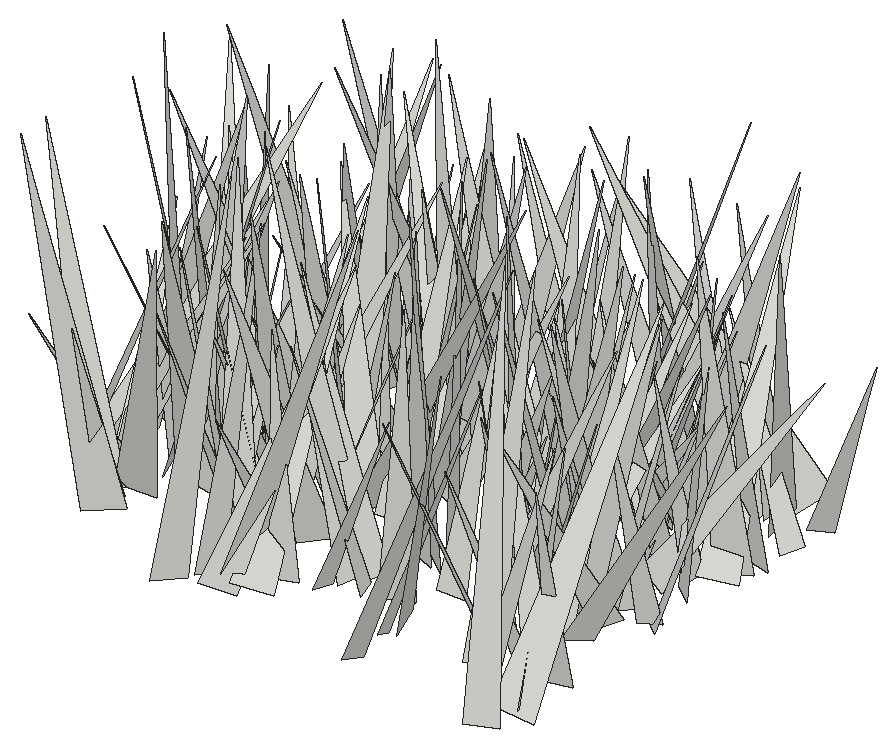
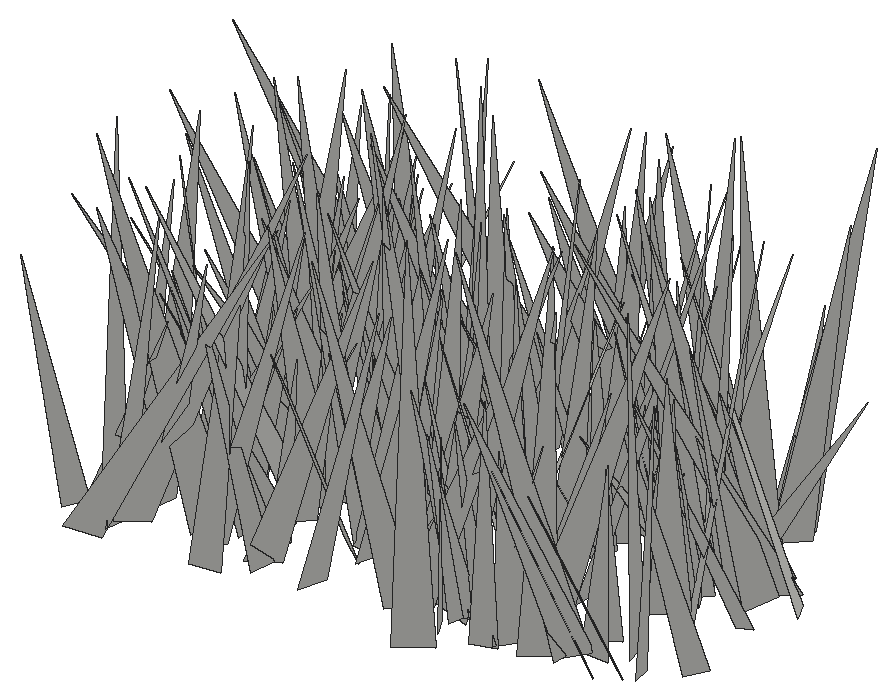
# SketchUp Ruby script. Lengths in inches.
U = 1.inch
M = Sketchup.active_model
def pt(a) = Geom::Point3d.new(a.map { |v| v * U })
def face(e, loops, mat)
  f = e.add_face(loops[0].map { |a| pt(a) })
  loops[1..].each { |l| e.add_face(l.map { |a| pt(a) }).erase! }
  f.material = f.back_material = mat if mat
  f
end
# faces: each face lists its corners as indices into pts; further lists are holes
def faces(e, pts, list, mat = nil) = list.each { |f| face(e, (f[0].is_a?(Array) ? f : [f]).map { |l| l.map { |i| pts[i] } }, mat) }
# xy, xz, yz: faces in a plane at the given z, y or x. An outline is a flat list of corners, or four numbers for a rectangle; further outlines are holes
def ring(l) = l.size == 4 ? [[l[0], l[1]], [l[2], l[1]], [l[2], l[3]], [l[0], l[3]]] : l.each_slice(2).to_a
def flat(e, list, mat, &to3) = list.each { |f| face(e, (f[0].is_a?(Array) ? f : [f]).map { |l| ring(l).map { |u, v| to3.(u, v) } }, mat) }
def xy(e, z, list, mat = nil) = flat(e, list, mat) { |x, y| [x, y, z] }
def xz(e, y, list, mat = nil) = flat(e, list, mat) { |x, z| [x, y, z] }
def yz(e, x, list, mat = nil) = flat(e, list, mat) { |y, z| [x, y, z] }
def lines(e, pts, list) = list.each { |a, b| e.add_line(pt(pts[a]), pt(pts[b])) }
# prism: a flat outline (further loops are holes) pulled along v
def prism(e, loops, v, mat = nil)
  f = face(e, loops, mat); d = Geom::Vector3d.new(v.map { |x| x * U })
  f.pushpull(f.normal.samedirection?(d) ? d.length : -d.length)
end
def box(e, o, s, mat = nil) = prism(e, [[o, [o[0] + s[0], o[1], o[2]], [o[0] + s[0], o[1] + s[1], o[2]], [o[0], o[1] + s[1], o[2]]]], [0, 0, s[2]], mat)
def at(x, y, z, deg = 0) = Geom::Transformation.translation(pt([x, y, z])) * Geom::Transformation.rotation(ORIGIN, Z_AXIS, deg.degrees)
def axes(o, x, y, z) = Geom::Transformation.new([*x, 0, *y, 0, *z, 0, *pt(o).to_a, 1])
def part(name) = M.definitions.add(name)
# library, detail: a bought-in or finely detailed component or shape, given as its bounding box
def library(name, o, s) = part(name).tap { |d| box(d.entities, o, s) }
def detail(e, o, s) = box(e.add_group.entities, o, s)
def put(e, d, t, mat = nil) = e.add_instance(d, t).tap { |i| i.material = mat if mat }
def group(e, t, mat = nil) = e.add_group.tap { |g| g.transformation = t; g.material = mat if mat }.entities
root = M.entities
c1 = part("fur_instance\#9")
p = [[0.8125,0,1.79],[0.67,-0.02,1.48],[0,-0.11,0],[0,0.11,0]]
faces(c1.entities,p,[[0,1,2,3]])
put(root,c1,axes([156.88,414.5625,-27.1],[4.55494,-1.38322,1.77977],[-1.90749,-4.50337,1.38185],[-1.20098,1.9065,4.55536]))
put(root,c1,axes([138.06,416.81,-27.1],[2.50523,-6.92108,2.84903],[-7.08461,-3.16179,-1.45116],[-2.41383,2.09672,7.21607]))
put(root,c1,axes([158.23,412.92,-27.1],[0.30584,8.28043,0.48557],[7.987,-0.4251,2.21855],[-2.2381,-0.38549,7.98355]))
put(root,c1,axes([151.5,417.05,-27.1],[6.22131,1.299,1.34326],[1.60809,-6.10017,-1.54868],[-0.95174,-1.81575,6.1639]))
put(root,c1,axes([158.52,416.99,-27.1],[1.07632,-4.38935,0.89904],[-4.4763,-1.09335,0.02097],[-0.19334,0.87825,4.51934]))
put(root,c1,axes([143.01,414.3,-27.1],[-6.71814,2.72987,2.53139],[2.23652,7.13443,-1.75826],[2.97626,0.8008,7.03521]))
put(root,c1,axes([155.51,417.1,-27.1],[-3.79986,-3.34827,0.10157],[-3.34083,3.7767,-0.4853],[-0.24505,0.43103,5.04126]))
put(root,c1,axes([137.81,417.57,-27.1],[2.72704,-3.27265,0.76108],[-3.17295,-2.83078,-0.80329],[-1.10537,0.05182,4.1835]))
put(root,c1,axes([138.07,418.58,-27.1],[2.36593,-6.95857,0.28973],[-6.83072,-2.25873,1.53056],[1.359,0.76137,7.18865]))
put(root,c1,axes([156.9,417.11,-27.1],[-0.5806,-4.0301,0.94816],[-3.96701,0.26756,-1.29192],[-1.18471,1.07913,3.86131]))
put(root,c1,axes([158.72,414.83,-27.1],[-4.5247,0.14497,1.56827],[-0.47946,4.4174,-1.79167],[1.5002,1.84904,4.15738]))
put(root,c1,axes([146.21,416.8,-27.1],[-1.45922,4.42701,2.15741],[4.90506,1.50733,0.22462],[0.43952,-2.12407,4.65589]))
put(root,c1,axes([144.89,415.73,-27.1],[7.47756,-1.51643,1.55812],[-1.8154,-7.42558,1.48539],[-1.19651,1.78955,7.48379]))
put(root,c1,axes([144.78,414.83,-27.1],[-3.66435,5.27166,1.90181],[4.6134,4.12758,-2.55233],[3.18179,0.08644,5.89097]))
put(root,c1,axes([151.63,413.93,-27.1],[7.3603,1.92647,1.4977],[1.22652,-7.03518,3.02165],[-2.10951,2.63124,6.98247]))
put(root,c1,axes([144.33,418.89,-27.1],[1.81992,-3.21241,0.00061],[-3.09433,-1.75321,-0.99152],[-0.86298,-0.48823,3.55649]))
put(root,c1,axes([143.84,415.58,-27.1],[-6.0255,1.4926,2.28597],[0.94971,6.33899,-1.63567],[2.5596,1.16168,5.98825]))
put(root,c1,axes([147.59,417.28,-27.1],[4.04534,-0.8517,0.30361],[-0.87788,-4.03293,0.38361],[-0.21657,0.43867,4.11619]))
put(root,c1,axes([158.59,414.24,-27.1],[-1.16046,8.00046,0.20395],[7.87345,1.17823,-1.41992],[1.43448,0.00519,7.95851]))
put(root,c1,axes([148.91,418.0625,-27.1],[-4.66141,-1.64687,0.68606],[-1.65466,4.70851,0.06011],[0.66704,0.1713,4.94341]))
put(root,c1,axes([145.32,419.77,-27.1],[2.99002,-5.93259,1.12286],[-5.76165,-3.17812,-1.449],[-1.8055,0.31717,6.48354]))
put(root,c1,axes([141.33,419.81,-27.1],[-4.0085,-3.44331,0.94309],[-3.06456,4.04605,1.74695],[1.83147,-0.76613,4.98725]))
put(root,c1,axes([150.23,418.15,-27.1],[2.8988,-5.16102,2.16058],[-5.5292,-3.01461,0.21733],[-0.85564,1.9958,5.91539]))
put(root,c1,axes([144.27,416.76,-27.1],[-5.43034,-1.89464,0.64767],[-1.9986,5.01546,-2.08529],[-0.12137,2.18018,5.36002]))
put(root,c1,axes([137.33,417.82,-27.1],[-5.93712,3.87569,1.72238],[4.1151,5.9813,0.72589],[1.02637,-1.56207,7.0529]))
put(root,c1,axes([151.37,415.99,-27.1],[4.47299,1.54799,0.88013],[1.09405,-4.26651,1.94385],[-1.40498,1.60599,4.31572]))
put(root,c1,axes([138.91,421.1,-27.1],[6.44625,-4.17663,0.34492],[-3.99481,-6.31514,-1.81045],[-1.26676,-1.33867,7.46462]))
put(root,c1,axes([137.73,419.21,-27.1],[-0.38653,-3.78857,0.47263],[-3.40937,0.1287,-1.7566],[-1.71837,0.59684,3.37891]))
put(root,c1,axes([155.375,416.58,-27.1],[-6.19625,3.45387,1.64148],[3.0912,6.3638,-1.72156],[2.25127,0.76815,6.88178]))
put(root,c1,axes([155.24,418.5625,-27.1],[-4.18009,-2.38384,1.39005],[-2.61185,4.23208,-0.59649],[0.8906,1.22265,4.77494]))
put(root,c1,axes([143.08,418.08,-27.1],[-2.11891,6.73628,2.3501],[7.12334,2.13432,0.30482],[0.39806,-2.33612,7.05509]))
put(root,c1,axes([143.9,418.87,-27.1],[-3.99562,-4.42007,1.47298],[-4.65768,3.83659,-1.12173],[0.11293,1.84803,5.85182]))
put(root,c1,axes([142.59,418.15,-27.1],[-0.05946,3.80591,1.08242],[3.88392,0.26301,-0.71143],[0.75616,-1.05166,3.7393]))
put(root,c1,axes([145.18,416.88,-27.1],[5.43487,-1.88004,3.06705],[-2.9758,-5.47185,1.91904],[-2.02138,3.00059,5.42123]))
put(root,c1,axes([148.13,418.53,-27.1],[-8.02945,1.44749,0.94959],[1.4539,8.08421,-0.0293],[0.93976,-0.13944,8.15883]))
put(root,c1,axes([154.01,420.71,-27.1],[0.47232,-5.02453,0.37853],[-5.03579,-0.45765,0.20889],[0.17316,0.39615,5.04235]))
put(root,c1,axes([156.79,417.9375,-27.1],[-1.63602,4.97918,0.62205],[4.87533,1.42244,1.43652],[-1.18757,-1.0199,5.04036]))
put(root,c1,axes([157.19,421.46,-27.1],[2.87484,-4.36178,0.57915],[-3.91954,-2.85297,-2.03053],[-1.99945,-0.67874,4.81319]))
put(root,c1,axes([145.75,415.57,-27.1],[-4.59589,5.78444,0.11594],[5.4804,4.40003,-2.28044],[1.8543,1.33244,7.02721]))
put(root,c1,axes([143.55,420.53,-27.1],[-0.33962,-4.53633,0.58104],[-4.49375,0.22275,-0.88758],[-0.84975,0.63509,4.46159]))
put(root,c1,axes([142.36,421.87,-27.1],[6.58115,-3.41587,1.26301],[-3.10443,-6.62563,-1.74311],[-1.90417,-1.00387,7.20703]))
put(root,c1,axes([148.61,419.01,-27.1],[-5.80532,1.01557,0.17125],[1.00882,5.80466,-0.22508],[0.20737,0.19232,5.88918]))
put(root,c1,axes([138.62,422.5625,-27.1],[-3.25593,-5.45811,0.05054],[-5.36708,3.21208,1.12765],[0.99394,-0.53501,6.25464]))
put(root,c1,axes([149.46,421.22,-27.1],[-3.95013,-6.45103,2.53754],[-6.55598,4.42551,1.04517],[2.25256,1.56763,7.49179]))
put(root,c1,axes([153.51,419.5,-27.1],[2.52048,5.79703,1.2985],[5.75928,-2.03853,-2.07834],[1.45681,-1.97061,5.96983]))
put(root,c1,axes([135.79,419.68,-27.1],[4.10268,4.53992,0.30052],[4.35228,-3.79801,-2.04106],[1.3262,-1.58032,5.76861]))
put(root,c1,axes([142.4,420.125,-27.1],[-2.65775,-2.55388,1.91088],[-2.80676,3.05414,0.17806],[1.51521,1.17784,3.68161]))
put(root,c1,axes([148.78,421.14,-27.1],[-1.6159,-6.90986,2.38073],[-7.13771,2.01606,1.00679],[1.57067,2.05292,7.0245]))
put(root,c1,axes([137.93,421.52,-27.1],[3.7662,-3.06911,1.25827],[-2.92554,-3.97067,-0.92842],[-1.56328,0.03677,4.76883]))
put(root,c1,axes([151.5,419.65,-27.1],[-0.63443,5.02312,1.44392],[5.17666,0.80438,-0.52377],[0.72032,-1.3566,5.03586]))
put(root,c1,axes([157.02,419.89,-27.1],[5.8068,-2.41673,0.19711],[-2.36119,-5.5195,1.88633],[0.55156,1.81463,6.0001]))
put(root,c1,axes([136.15,420.29,-27.1],[3.52755,5.08967,0.59914],[4.90233,-3.13928,-2.19532],[1.49362,-1.71683,5.79042]))
put(root,c1,axes([139.86,420.15,-27.1],[1.56528,5.39191,1.82425],[5.61252,-1.77733,0.43748],[-0.9488,-1.61836,5.59744]))
put(root,c1,axes([155.9,421.4,-27.1],[-2.90009,-5.61636,1.60668],[-5.82709,2.65472,-1.23809],[-0.41218,1.98605,6.19848]))
put(root,c1,axes([153.88,421.9375,-27.1],[4.89387,1.35478,0.49174],[1.44124,-4.60961,-1.64362],[-0.00784,-1.71558,4.80457]))
put(root,c1,axes([146.14,420.9,-27.1],[3.85266,4.81198,3.39076],[5.17881,-4.69725,0.78179],[-2.79863,-2.06788,6.11449]))
put(root,c1,axes([155.28,423.59,-27.1],[3.26606,-6.16963,0.62937],[-6.14796,-3.31446,-0.58694],[-0.81426,0.27855,6.95607]))
put(root,c1,axes([138.24,423.05,-27.1],[-6.05203,-3.65216,2.90127],[-3.20675,6.70926,1.75646],[3.38709,-0.1736,6.84691]))
put(root,c1,axes([142.83,423.29,-27.1],[-3.8372,-2.33717,0.79383],[-2.01321,3.81242,1.493],[1.42812,-0.90538,4.23762]))
put(root,c1,axes([153.32,421.24,-27.1],[-6.66859,-2.01923,2.71074],[-2.32845,7.09045,-0.44648],[2.45024,1.24248,6.95328]))
put(root,c1,axes([158.25,422.43,-27.1],[1.30026,-4.12004,1.09762],[-4.18224,-1.45572,-0.50983],[-0.82967,0.8811,4.29016]))
put(root,c1,axes([136.82,419.54,-27.1],[-2.17484,4.53028,0.06229],[4.50087,2.16823,-0.54601],[0.51907,0.1805,4.99552]))
put(root,c1,axes([133.94,421.53,-27.1],[5.98281,3.47845,0.55141],[3.51313,-5.81778,-1.41742],[0.2481,-1.50052,6.77381]))
put(root,c1,axes([137.92,420.65,-27.1],[6.78168,2.91502,1.19431],[2.8839,-6.88568,0.43057],[-1.26762,-0.07012,7.36906]))
put(root,c1,axes([155.07,423.51,-27.1],[1.17594,-4.92519,0.34785],[-4.93492,-1.18388,-0.07952],[-0.1583,0.31979,5.06301]))
put(root,c1,axes([139.65,421.64,-27.1],[3.10895,3.01642,1.49943],[3.22004,-3.26039,-0.11754],[-0.98914,-1.13301,4.33019]))
put(root,c1,axes([151.19,422.47,-27.1],[2.68666,-2.71893,0.01615],[-2.65256,-2.616,0.85524],[0.59729,0.61233,3.72549]))
put(root,c1,axes([153.03,421.77,-27.1],[3.30994,1.56111,0.94089],[1.62723,-3.40964,-0.0672],[-0.82125,-0.46405,3.659]))
put(root,c1,axes([140.05,421.42,-27.1],[3.54809,3.00738,1.07129],[3.07779,-3.64774,0.04651],[-0.84804,-0.65624,4.65093]))
put(root,c1,axes([142.13,422.45,-27.1],[2.86459,-3.18276,1.27512],[-3.34476,-2.95943,0.1272],[-0.754,1.03614,4.28015]))
put(root,c1,axes([153.55,422.21,-27.1],[-3.32572,-4.76152,1.64129],[-5.0351,3.09772,-1.21581],[-0.11678,2.03921,5.67929]))
put(root,c1,axes([141.63,420.7,-27.1],[-0.67642,4.08917,0.12939],[3.98053,0.62749,0.97839],[-0.94522,-0.2838,4.0276]))
put(root,c1,axes([137.56,422.21,-27.1],[3.65064,-1.60023,0.53489],[-1.66152,-3.63138,0.47591],[-0.29361,0.65299,3.95745]))
put(root,c1,axes([142.9,421.66,-27.1],[0.16923,4.07191,1.2027],[4.12697,0.12503,-1.00402],[0.99752,-1.2081,3.94982]))
put(root,c1,axes([155.28,422.42,-27.1],[0.56131,-6.10589,2.64479],[-6.41112,0.21442,1.85565],[1.78167,2.69518,5.8441]))
put(root,c1,axes([138.05,421.36,-27.1],[3.6249,6.4726,3.15784],[6.5149,-4.45394,1.65071],[-3.06961,-1.8095,7.23254]))
put(root,c1,axes([156,420.01,-27.1],[0.77683,6.56918,0.32302],[6.56801,-0.79193,0.30978],[-0.34589,-0.28401,6.60769]))
put(root,c1,axes([157.04,422.73,-27.1],[-1.11932,5.12608,2.18052],[5.30702,0.30525,2.00664],[-1.6932,-2.43194,4.84799]))
put(root,c1,axes([135.375,422.09,-27.1],[6.77248,-2.83159,1.61361],[-3.13932,-6.6674,1.47599],[-0.87537,2.00399,7.19067]))
put(root,c1,axes([137.61,423.14,-27.1],[5.01911,-5.50348,2.14134],[-5.83765,-5.04831,0.7082],[-0.89193,2.07156,7.41473]))
put(root,c1,axes([140.43,425.61,-27.1],[-7.65526,-2.65251,1.50577],[-2.23878,7.64939,2.09305],[2.07148,-1.53532,7.82675]))
put(root,c1,axes([136.4,424.68,-27.1],[-5.36571,-5.00333,1.81378],[-4.95811,5.63559,0.87824],[1.93398,0.5664,7.28374]))
put(root,c1,axes([145.28,422.62,-27.1],[7.55011,-1.58138,0.22082],[-1.59514,-7.42262,1.38345],[0.0711,1.39915,7.58887]))
put(root,c1,axes([135.15,420.88,-27.1],[0.81957,8.13408,0.73803],[7.68253,-0.51597,-2.84467],[2.77248,-0.97476,7.66439]))
put(root,c1,axes([152.63,424.03,-27.1],[7.05562,-2.47543,1.6862],[-2.53392,-7.23407,-0.01726],[-1.59697,0.54154,7.47725]))
put(root,c1,axes([152.8,424.64,-27.1],[2.44609,-6.94499,1.47158],[-6.99231,-2.08787,1.76924],[1.22722,1.94671,7.14745]))
put(root,c1,axes([152.75,420.76,-27.1],[1.27817,7.72916,0.81529],[7.27012,-1.48113,2.64386],[-2.74773,-0.32349,7.37453]))
put(root,c1,axes([149.71,421.92,-27.1],[-6.21182,-1.68937,2.27799],[-2.42044,6.01654,-2.13837],[1.47806,2.75267,6.07191]))
put(root,c1,axes([135.25,423.45,-27.1],[2.3418,4.95634,1.60959],[5.19702,-2.35112,-0.32146],[-0.38351,-1.59595,5.4723]))
put(root,c1,axes([141.39,425.84,-27.1],[5.68928,-3.36377,1.44998],[-3.11585,-5.85243,-1.35122],[-1.92583,-0.46842,6.46971]))
put(root,c1,axes([147.45,421.84,-27.1],[5.41894,2.39891,1.8987],[1.67708,-5.5593,2.23748],[-2.55876,1.4367,5.48756]))
put(root,c1,axes([154.06,422.74,-27.1],[2.83544,5.2975,1.05869],[5.3487,-2.92083,0.29014],[-0.75876,-0.79328,6.00159]))
put(root,c1,axes([138.41,422.25,-27.1],[3.83996,1.68055,0.1423],[1.49178,-3.54944,1.66307],[-0.78682,1.47206,3.84756]))
put(root,c1,axes([146.5625,422.59,-27.1],[-1.26821,6.79621,1.34265],[6.86908,1.41065,-0.65215],[0.89826,-1.19212,6.8827]))
put(root,c1,axes([156.75,422.13,-27.1],[2.63197,4.07891,0.20518],[3.86496,-2.5665,1.44292],[-1.31973,0.61842,4.63495]))
put(root,c1,axes([138.45,423.51,-27.1],[-1.05429,4.67357,0.99792],[4.75005,0.91265,0.74413],[-0.52453,-1.12891,4.73287]))
put(root,c1,axes([137.33,422.9,-27.1],[3.31155,2.43431,1.59522],[1.82743,-3.61986,1.73033],[-2.2652,0.63849,3.72802]))
put(root,c1,axes([134.72,423.6875,-27.1],[1.36791,4.73736,0.76135],[4.55305,-1.0318,-1.76027],[1.51392,-1.17738,4.60599]))
put(root,c1,axes([152.19,423.78,-27.1],[3.72107,-3.56028,1.90501],[-4.03778,-3.30047,1.71878],[-0.03061,2.5656,4.85467]))
put(root,c1,axes([153.92,424.24,-27.1],[-4.56501,-1.69942,1.47091],[-1.97129,4.62695,-0.77219],[1.07964,1.26263,4.80947]))
put(root,c1,axes([149.29,425.37,-27.1],[1.54528,-3.8993,0.59524],[-3.77652,-1.27799,1.43226],[1.13873,1.05307,3.94222]))
put(root,c1,axes([158.62,422.13,-27.1],[3.88995,3.95886,0.07672],[3.75671,-3.72392,1.68217],[-1.25122,1.12695,5.2891]))
put(root,c1,axes([146.85,424.81,-27.1],[7.17764,0.6661,2.04171],[0.73913,-7.45363,-0.1667],[-2.01642,-0.36113,7.20655]))
put(root,c1,axes([147.49,424.7,-27.1],[1.43912,5.66343,2.07225],[5.60003,-0.46439,-2.61988],[2.23794,-2.47985,5.22319]))
put(root,c1,axes([155.02,425.85,-27.1],[-0.84306,-4.44176,0.86686],[-4.52258,0.85891,0.00263],[0.16427,0.85115,4.52106]))
put(root,c1,axes([154.27,422.73,-27.1],[-0.54715,4.89077,0.10405],[4.53126,0.54616,-1.84371],[1.84341,0.10915,4.56287]))
put(root,c1,axes([156.3125,425.86,-27.1],[0.08099,-5.17118,1.20761],[-5.27072,-0.22549,-0.61212],[-0.64729,1.18913,5.13546]))
put(root,c1,axes([143.2,423.86,-27.1],[3.15167,2.15202,0.19961],[2.1362,-3.1554,0.29004],[-0.32814,0.12762,3.80527]))
put(root,c1,axes([148.56,427.7,-27.1],[-2.04467,-7.63412,0.65301],[-7.56547,2.11851,1.07815],[1.21235,0.345,7.82931]))
put(root,c1,axes([152.45,426.04,-27.1],[-1.50167,-7.67594,2.08534],[-7.92089,1.24921,-1.10571],[-0.72669,2.24569,7.7429]))
put(root,c1,axes([142.38,427.95,-27.1],[-4.33714,-4.09832,0.0827],[-3.81397,4.0787,2.10515],[1.50223,-1.4771,5.58349]))
put(root,c1,axes([143.84,424.31,-27.1],[-4.18107,4.06515,1.12452],[4.17237,4.21812,0.26475],[0.61747,-0.97641,5.82552]))
put(root,c1,axes([157.47,425.88,-27.1],[-4.17455,0.44699,1.70239],[0.80041,4.38471,0.81146],[1.56757,-1.04848,4.11925]))
put(root,c1,axes([154.5,425.29,-27.1],[-3.00148,-2.27694,0.1564],[-2.20162,2.82047,-1.1898],[-0.60148,1.03841,3.57459]))
put(root,c1,axes([153.21,425.66,-27.1],[6.75875,-1.16964,0.00047],[-1.16859,-6.75255,0.29358],[0.0496,0.28936,6.85293]))
put(root,c1,axes([142.48,425.71,-27.1],[2.08402,3.38406,1.47593],[3.68931,-1.84524,-0.97848],[0.13865,-1.76538,3.85196]))
put(root,c1,axes([151.42,425.42,-27.1],[-2.68831,3.38264,1.06218],[3.54497,2.54168,0.8778],[-0.06058,-1.37662,4.23069]))
put(root,c1,axes([141.0625,423.7,-27.1],[2.76171,5.55128,0.00194],[5.48471,-2.72826,-0.95829],[0.85713,-0.42855,6.1258]))
put(root,c1,axes([157.875,424.77,-27.1],[3.73887,4.62596,1.90486],[4.75099,-4.02818,0.45718],[-1.5672,-1.17533,5.9304]))
put(root,c1,axes([138.22,424.52,-27.1],[-1.29816,5.29172,0.79515],[5.27739,1.13069,1.0911],[-0.88529,-1.01932,5.33826]))
put(root,c1,axes([146.02,426.78,-27.1],[-0.11111,-7.60969,2.49454],[-7.52897,0.94928,2.56048],[2.72852,2.30953,7.16685]))
put(root,c1,axes([156.36,424.89,-27.1],[1.31269,5.55847,0.82299],[4.82858,-0.68361,-3.08457],[2.8738,-1.39037,4.80678]))
put(root,c1,axes([153.85,424.06,-27.1],[-1.09311,5.26549,0.63584],[5.05113,1.23151,-1.51458],[1.61731,-0.28736,5.16007]))
put(root,c1,axes([156.67,427.15,-27.1],[-1.81586,-4.37557,0.34615],[-4.20637,1.62778,-1.48984],[-1.25376,0.87607,4.49704]))
put(root,c1,axes([158.36,427.03,-27.1],[-2.64442,5.36733,3.49605],[6.32318,2.79183,0.49668],[1.02376,-3.3795,5.96276]))
put(root,c1,axes([142.53,425.34,-27.1],[-5.26533,5.42334,2.66225],[5.51698,5.75546,-0.81326],[2.46233,-1.29842,7.51498]))
put(root,c1,axes([151.46,425.24,-27.1],[-5.91196,3.62871,1.99788],[3.48429,6.23911,-1.02156],[2.24027,-0.12769,6.86114]))
put(root,c1,axes([137.45,424.53,-27.1],[-4.42637,5.44798,0.10976],[5.44745,4.42761,-0.08267],[0.13338,-0.03304,7.019]))
put(root,c1,axes([151.6875,427.3125,-27.1],[-3.71371,1.13934,1.58672],[1.47505,3.87017,0.67337],[1.28063,-1.15373,3.82574]))
put(root,c1,axes([149.36,426.73,-27.1],[7.16515,0.1083,1.44204],[0.09788,-7.3087,0.06254],[-1.44279,0.042,7.1657]))
put(root,c1,axes([155.14,426.0625,-27.1],[-1.55107,4.41542,0.77186],[4.34501,1.28043,1.40671],[-1.10114,-1.16708,4.46351]))
put(root,c1,axes([134.03,427.3,-27.1],[2.085,-4.49657,0.98747],[-4.39792,-1.62495,1.88661],[1.36107,1.63764,4.58334]))
put(root,c1,axes([141.14,427.05,-27.1],[-1.13244,4.66111,1.93868],[4.91983,0.57378,1.4943],[-1.13125,-2.17064,4.55801]))
put(root,c1,axes([158.625,428.03,-27.1],[-1.20745,-5.31811,1.49773],[-5.50418,1.29079,0.14593],[0.47907,1.42653,5.45151]))
put(root,c1,axes([139.22,429.8,-27.1],[6.38115,-3.67921,0.2036],[-3.55943,-6.25987,-1.56256],[-0.95316,-1.25481,7.1982]))
put(root,c1,axes([136.625,427.36,-27.1],[-5.78196,-1.74059,3.08913],[-1.82129,6.52793,0.26926],[3.04225,0.59997,6.03227]))
put(root,c1,axes([146.49,426.25,-27.1],[0.66704,7.88186,2.68055],[8.14998,-1.16705,1.40349],[-1.69907,-2.50365,7.78452]))
put(root,c1,axes([155.61,425.22,-27.1],[3.29969,3.36632,0.10349],[3.25213,-3.22241,1.12716],[-0.87548,0.71745,4.57707]))
put(root,c1,axes([142.9375,426.2,-27.1],[1.28068,6.67783,2.12971],[6.86225,-1.63556,1.00185],[-1.42781,-1.87102,6.72532]))
put(root,c1,axes([146.75,425.95,-27.1],[-4.59485,5.55244,0.46156],[5.5505,4.50971,1.00485],[-0.48434,-0.99407,7.1367]))
put(root,c1,axes([140.03,428.42,-27.1],[-0.48012,-7.554,2.16495],[-7.6037,-0.10085,-2.03814],[-1.98335,2.21526,7.28968]))
put(root,c1,axes([146.01,429.15,-27.1],[4.30794,-3.29071,0.86204],[-3.07513,-4.36194,-1.28347],[-1.45447,-0.52435,5.26686]))
put(root,c1,axes([144,425.47,-27.1],[3.8094,4.08661,1.06154],[3.80016,-3.94157,1.53675],[-1.84012,0.32005,5.37125]))
put(root,c1,axes([137.83,427.35,-27.1],[1.56835,-2.82264,1.69633],[-3.20586,-1.73838,0.07137],[-0.75322,1.52161,3.2283]))
put(root,c1,axes([155.58,426.2,-27.1],[3.89268,2.82638,0.90518],[2.67493,-3.98806,0.94914],[-1.28551,0.26015,4.71599]))
put(root,c1,axes([152.82,427.61,-27.1],[2.65844,-2.5721,0.0216],[-2.2994,-2.3625,1.67773],[1.15278,1.21916,3.2967]))
put(root,c1,axes([144.21,428.93,-27.1],[4.56733,-2.95407,1.62637],[-2.80415,-4.84794,-0.93072],[-1.87305,0.05455,5.35918]))
put(root,c1,axes([135.47,428.61,-27.1],[-4.30625,-1.78107,2.16646],[-1.55574,4.81995,0.87021],[2.33354,-0.07334,4.57807]))
put(root,c1,axes([148.45,426.97,-27.1],[-1.13275,3.97734,1.11963],[3.98013,1.3621,-0.81189],[1.10966,-0.82546,4.05502]))
put(root,c1,axes([152.58,425.36,-27.1],[-6.84761,2.51212,1.52779],[1.98246,6.80446,-2.30302],[2.17135,1.70976,6.92074]))
put(root,c1,axes([140.39,429.59,-27.1],[7.09602,-3.54407,1.49132],[-3.45875,-7.25092,-0.77408],[-1.67974,-0.04148,7.89397]))
put(root,c1,axes([148.15,427.81,-27.1],[-7.39383,1.79038,1.19471],[1.82356,7.48136,0.07416],[1.14343,-0.35412,7.60715]))
put(root,c1,axes([142.66,428.93,-27.1],[4.32257,0.5968,0.21737],[0.63053,-4.21214,-0.97382],[-0.07654,-0.99484,4.25352]))
put(root,c1,axes([153.93,428.57,-27.1],[2.87262,5.81566,3.24646],[6.49078,-3.23727,0.05584],[-1.49368,-2.88298,6.48619]))
put(root,c1,axes([144.61,430.18,-27.1],[-1.86183,-7.54983,1.10161],[-7.50699,1.61006,-1.65309],[-1.3633,1.44488,7.59827]))
put(root,c1,axes([143.7,429.27,-27.1],[-0.98581,-7.65367,2.64082],[-7.9173,0.35473,-1.92744],[-1.69382,2.79641,7.47232]))
put(root,c1,axes([142,429,-27.1],[-3.00946,-2.45302,0.73779],[-2.54129,3.00205,-0.38468],[0.32167,0.76736,3.86344]))
put(root,c1,axes([151.49,429.03,-27.1],[1.53479,-3.08573,1.52348],[-3.30012,-1.79268,-0.30636],[-0.97569,1.2095,3.43271]))
put(root,c1,axes([138.42,428.93,-27.1],[7.76844,-0.71206,0.72464],[-0.74639,-7.79129,0.34557],[-0.68922,0.41169,7.79335]))
put(root,c1,axes([157.37,431.02,-27.1],[7.02659,-0.33713,1.59],[0.09653,-6.95626,-1.90152],[-1.62247,-1.87389,6.7728]))
put(root,c1,axes([141.45,429.9,-27.1],[1.4619,-3.63585,0.57448],[-3.60479,-1.28901,1.01518],[0.74496,0.89757,3.78497]))
put(root,c1,axes([152.41,428.58,-27.1],[3.65176,6.04586,1.11201],[6.02251,-3.25936,-2.05677],[1.23222,-1.98709,6.75703]))
put(root,c1,axes([152.82,429.16,-27.1],[5.19271,0.37939,0.34653],[0.38191,-5.20401,-0.02543],[-0.34375,-0.05067,5.20649]))
put(root,c1,axes([158.19,426.33,-27.1],[-3.4412,6.39637,0.09759],[6.32165,3.41718,-1.06042],[0.97968,0.41743,7.18546]))
put(root,c1,axes([152.48,426.57,-27.1],[7.12213,3.78972,1.00867],[3.4176,-7.02352,2.25704],[-1.92338,1.55314,7.74548]))
put(root,c1,axes([156.5,431.17,-27.1],[-7.92246,2.32052,1.49756],[2.68865,7.5204,2.57051],[0.63138,-2.90715,7.84491]))
put(root,c1,axes([152.32,432.22,-27.1],[-1.3783,-7.92591,0.91068],[-7.76861,1.54372,1.6777],[1.81604,0.58822,7.86798]))
put(root,c1,axes([137.57,428.64,-27.1],[-1.32199,4.73147,0.88748],[4.77716,1.17578,0.84759],[-0.59431,-1.0737,4.83901]))
put(root,c1,axes([150.99,430.57,-27.1],[-5.87282,3.13064,1.60123],[3.47052,5.66214,1.65846],[0.56601,-2.23474,6.44519]))
put(root,c1,axes([153.12,430.85,-27.1],[-6.41083,1.14128,1.69671],[1.48537,6.43646,1.28286],[1.40536,-1.59673,6.38401]))
put(root,c1,axes([136.06,429.0625,-27.1],[2.47782,3.1575,0.0552],[3.13992,-2.45577,-0.47176],[0.33732,-0.3344,3.98583]))
put(root,c1,axes([158.9375,429.65,-27.1],[-4.27711,1.68369,0.0136],[1.68167,4.26988,0.26227],[-0.08344,-0.24902,4.58909]))
put(root,c1,axes([145.12,430.09,-27.1],[-0.35143,6.05342,2.99786],[6.31844,1.35633,-1.99808],[2.38924,-2.69649,5.72495]))
put(root,c1,axes([153.92,429.6875,-27.1],[6.10397,-4.61293,1.81963],[-4.95361,-5.80478,1.9013],[-0.22786,2.62185,7.41098]))
put(root,c1,axes([141.15,430.45,-27.1],[1.68942,-4.24341,1.91691],[-4.60334,-1.82876,0.00876],[-0.70022,1.78447,4.56734]))
put(root,c1,axes([143.02,429.38,-27.1],[3.50267,-1.34823,2.1537],[-1.97697,-3.75014,0.86764],[-1.59615,1.68627,3.65152]))
put(root,c1,axes([143.03,432.04,-27.1],[3.4393,-6.56896,1.063],[-6.65437,-3.3911,0.57422],[0.02233,1.20797,7.39258]))
put(root,c1,axes([143.21,430.33,-27.1],[3.08289,1.97486,1.70839],[2.08981,-3.45082,0.21788],[-1.56569,-0.71742,3.6547]))
put(root,c1,axes([142.81,429.25,-27.1],[-1.16488,5.07104,1.08343],[5.11451,1.30667,-0.61696],[0.85504,-0.90739,5.16641]))
put(root,c1,axes([150.79,430.89,-27.1],[5.32067,-0.59583,0.38531],[-0.58759,-5.33383,-0.13414],[-0.39777,-0.09079,5.35224]))
put(root,c1,axes([149.07,427.98,-27.1],[2.7978,5.22834,0.27095],[4.99402,-2.75746,1.64099],[-1.57121,0.54549,5.69828]))
put(root,c1,axes([148.62,430.78,-27.1],[-6.00997,1.04438,1.22572],[1.13938,6.10462,0.38513],[1.13796,-0.59647,6.08787]))
put(root,c1,axes([156.42,429.64,-27.1],[-6.22467,1.67352,0.58559],[1.62437,6.23957,-0.56507],[0.71064,0.39649,6.42089]))
put(root,c1,axes([158.81,431.39,-27.1],[3.25053,-3.28963,0.28157],[-3.26975,-3.15258,0.91484],[0.45796,0.84053,4.53329]))
put(root,c1,axes([157.35,432.86,-27.1],[-6.27712,3.42033,1.55819],[3.73626,5.34865,3.31076],[-0.40863,-3.63622,6.33559]))
put(root,c1,axes([156.74,431.54,-27.1],[5.59524,-0.57904,3.08549],[-0.36766,-6.38318,-0.53118],[-3.11775,-0.28642,5.59999]))
put(root,c1,axes([137.09,429.55,-27.1],[2.95968,3.81178,0.17357],[3.80838,-2.96454,0.16477],[-0.23661,-0.0359,4.82309]))
put(root,c1,axes([138.15,428.95,-27.1],[-2.51338,5.74575,1.01303],[5.46798,2.70448,-1.77311],[2.03497,-0.17044,6.01555]))
